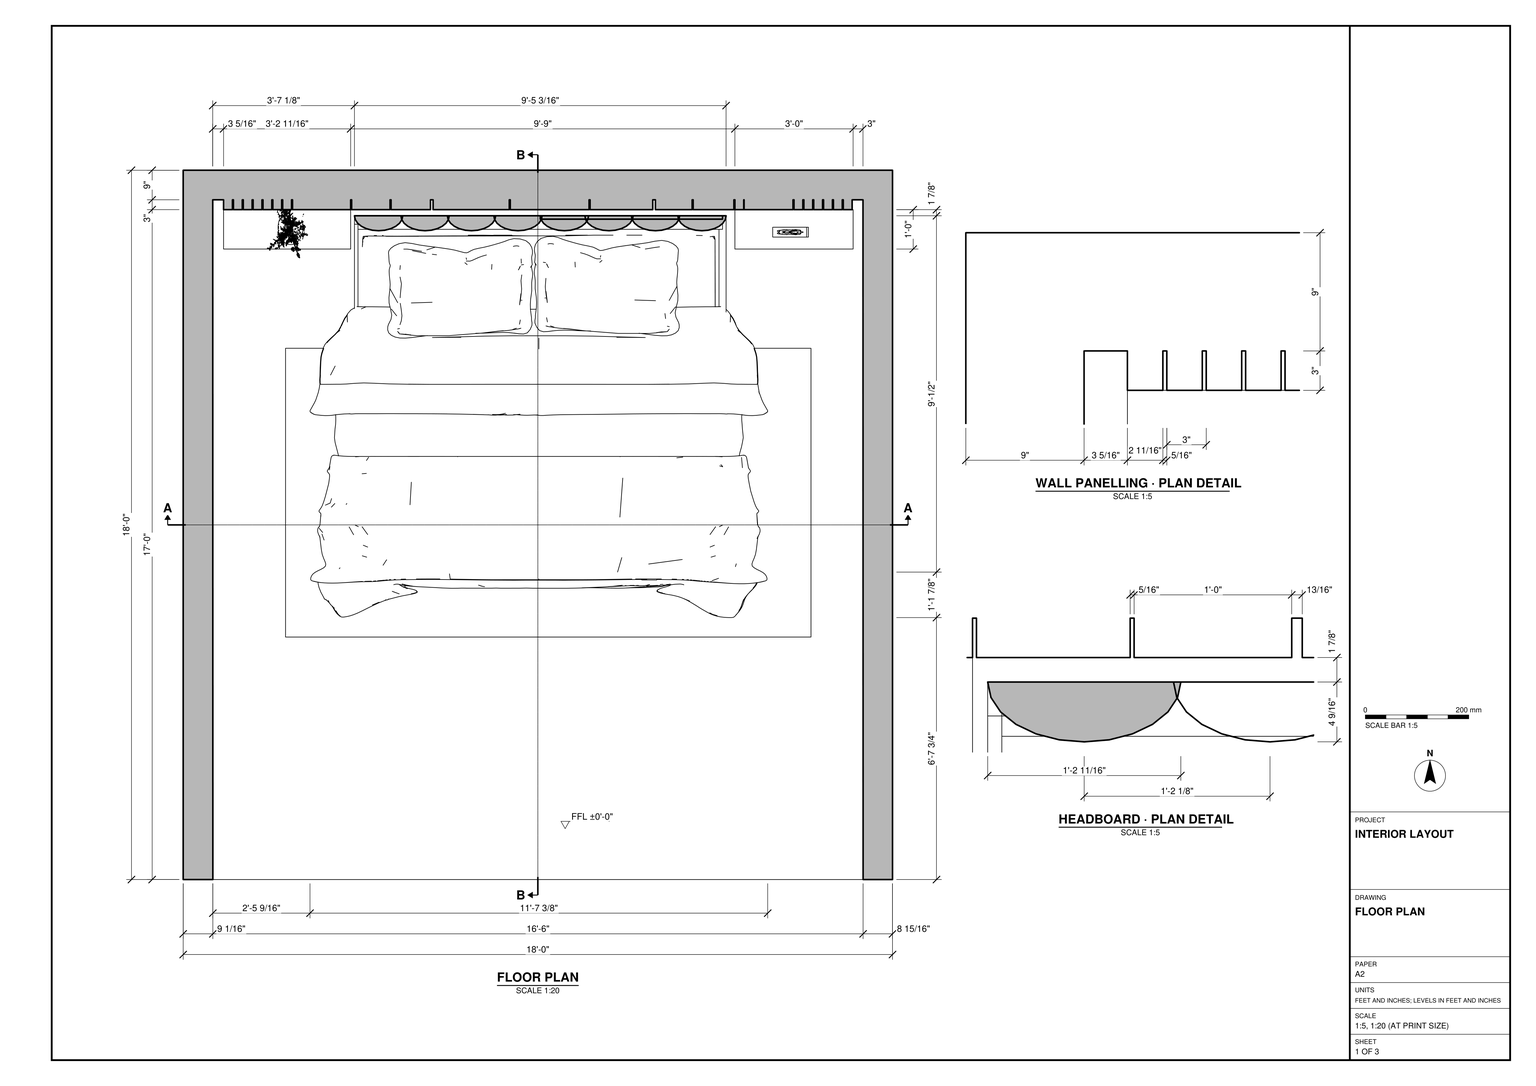
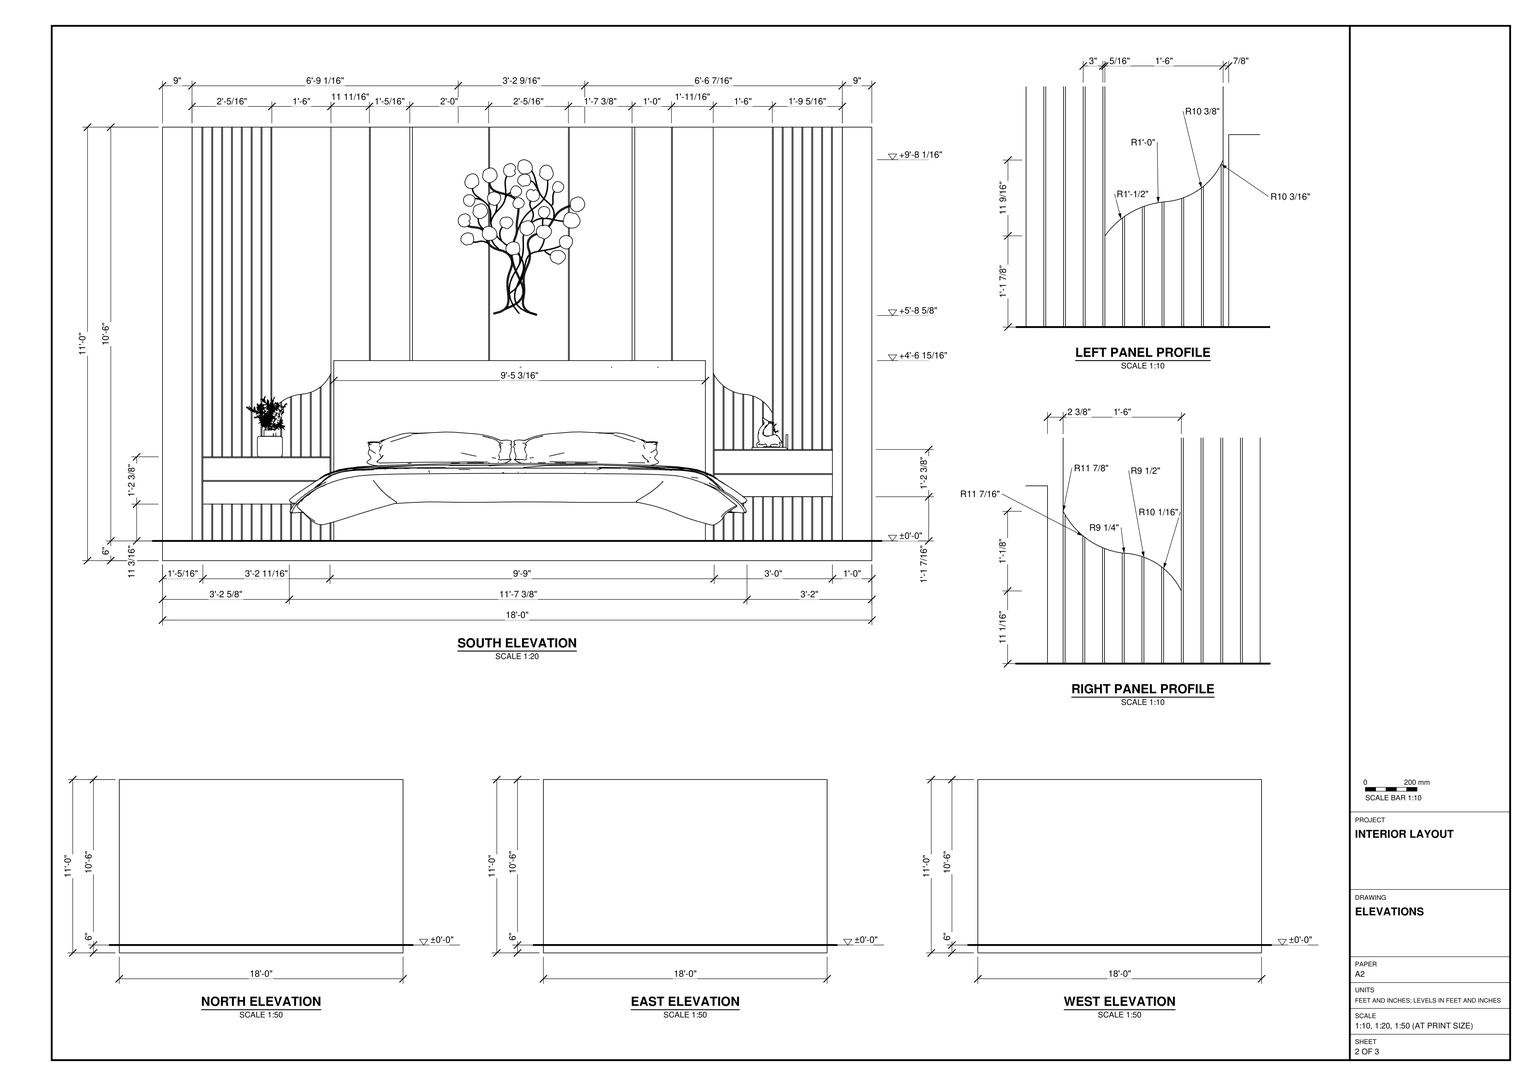
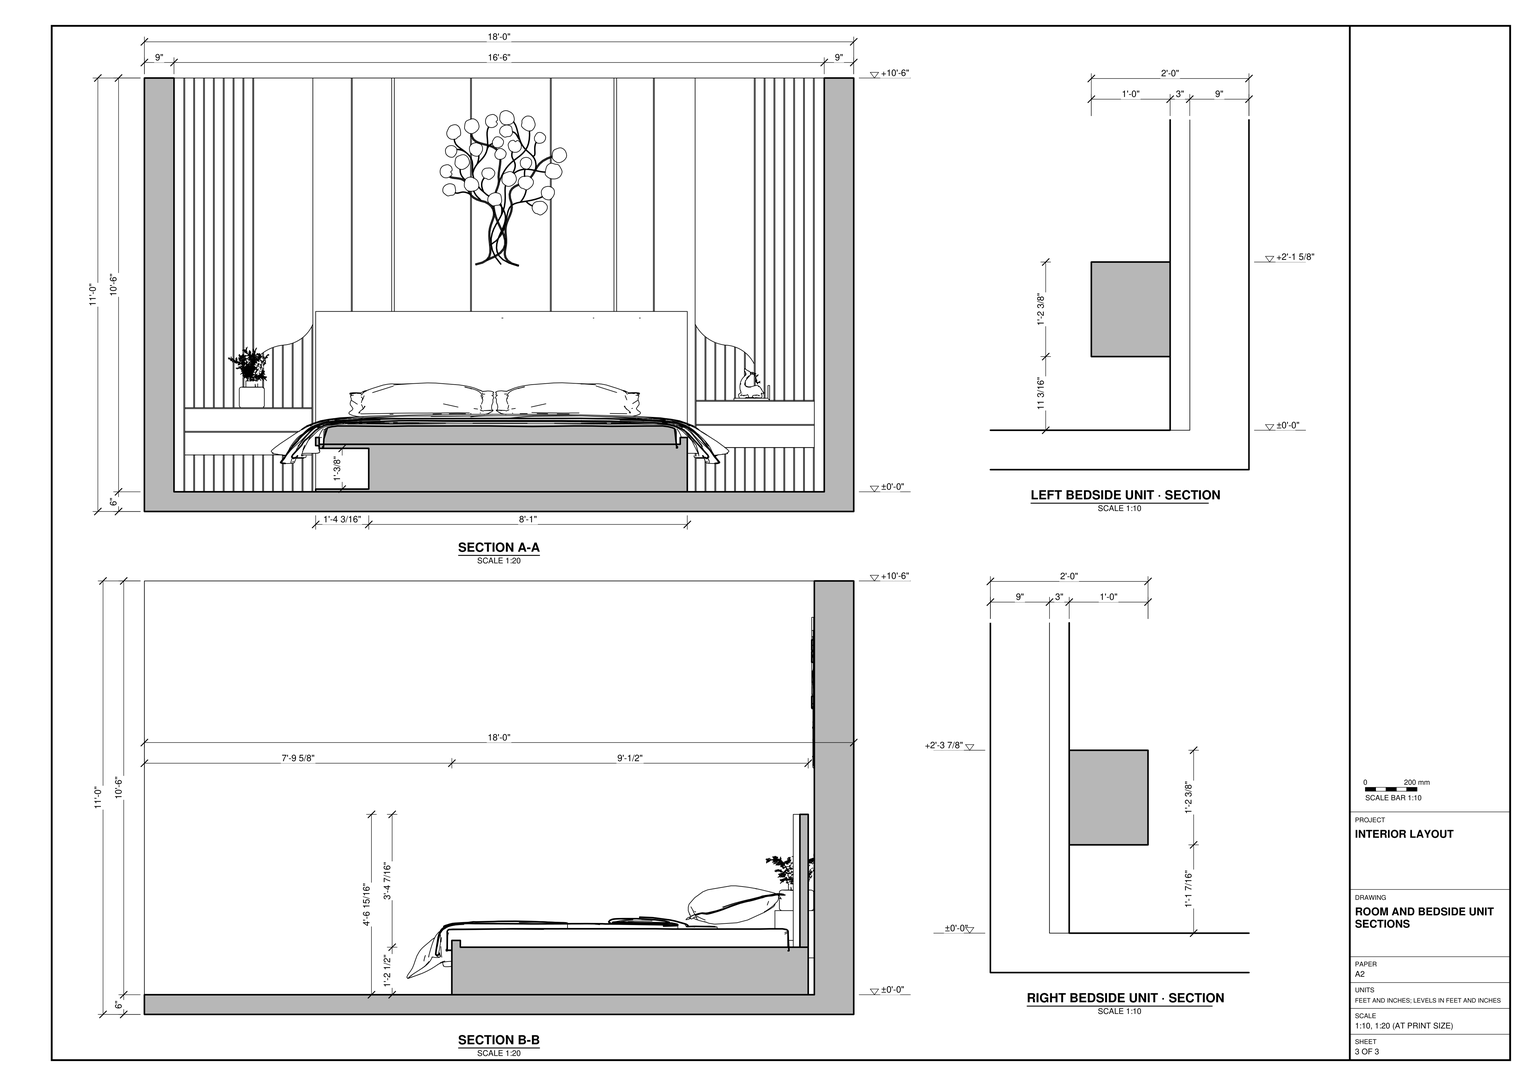
Build the bedroom in SketchUp from task_files/diagram_01.pdf. Work in feet and inches. The room measures 18'-0" by 18'-0" overall and is 11'-0" high from the underside of the floor slab to the wall tops. Set the finished floor at ±0'-0". Model the 6" slab and the three enclosing walls at the thicknesses shown, leaving the side opposite the headboard open as drawn.

Centre the platform bed against the back wall, with the mattress, pillows and covers arranged as in plan. Place the rectangular rug beneath the bed so that it extends beyond the sides and foot. Use the headboard plan detail to form the rounded sections across its face. Behind it, model the broad vertical panels in the middle of the wall and the closely spaced strips toward the ends. Follow the separate left and right profiles where the strip tops curve beside the headboard.

Fit a floating bedside unit on either side of the bed. Use the bedside sections for their projection and mounting heights; the right unit sits slightly higher than the left. Place the wall decoration above the headboard and the small objects on the bedside units as shown. Decor and loose items may be any suitable library components. Keep the walls, slab and each furniture or joinery piece in separate groups or components, and use components for repeated parts. Save one SketchUp model as output_files/bedroom_with_a_panelled_headboard_wall.skp.

# SketchUp Ruby script. Lengths in inches.
U = 1.inch
M = Sketchup.active_model
def pt(a) = Geom::Point3d.new(a.map { |v| v * U })
def face(e, loops, mat)
  f = e.add_face(loops[0].map { |a| pt(a) })
  loops[1..].each { |l| e.add_face(l.map { |a| pt(a) }).erase! }
  f.material = f.back_material = mat if mat
  f
end
# faces: each face lists its corners as indices into pts; further lists are holes
def faces(e, pts, list, mat = nil) = list.each { |f| face(e, (f[0].is_a?(Array) ? f : [f]).map { |l| l.map { |i| pts[i] } }, mat) }
# xy, xz, yz: faces in a plane at the given z, y or x. An outline is a flat list of corners, or four numbers for a rectangle; further outlines are holes
def ring(l) = l.size == 4 ? [[l[0], l[1]], [l[2], l[1]], [l[2], l[3]], [l[0], l[3]]] : l.each_slice(2).to_a
def flat(e, list, mat, &to3) = list.each { |f| face(e, (f[0].is_a?(Array) ? f : [f]).map { |l| ring(l).map { |u, v| to3.(u, v) } }, mat) }
def xy(e, z, list, mat = nil) = flat(e, list, mat) { |x, y| [x, y, z] }
def xz(e, y, list, mat = nil) = flat(e, list, mat) { |x, z| [x, y, z] }
def yz(e, x, list, mat = nil) = flat(e, list, mat) { |y, z| [x, y, z] }
def lines(e, pts, list) = list.each { |a, b| e.add_line(pt(pts[a]), pt(pts[b])) }
# prism: a flat outline (further loops are holes) pulled along v
def prism(e, loops, v, mat = nil)
  f = face(e, loops, mat); d = Geom::Vector3d.new(v.map { |x| x * U })
  f.pushpull(f.normal.samedirection?(d) ? d.length : -d.length)
end
def box(e, o, s, mat = nil) = prism(e, [[o, [o[0] + s[0], o[1], o[2]], [o[0] + s[0], o[1] + s[1], o[2]], [o[0], o[1] + s[1], o[2]]]], [0, 0, s[2]], mat)
def at(x, y, z, deg = 0) = Geom::Transformation.translation(pt([x, y, z])) * Geom::Transformation.rotation(ORIGIN, Z_AXIS, deg.degrees)
def axes(o, x, y, z) = Geom::Transformation.new([*x, 0, *y, 0, *z, 0, *pt(o).to_a, 1])
def part(name) = M.definitions.add(name)
# library, detail: a bought-in or finely detailed component or shape, given as its bounding box
def library(name, o, s) = part(name).tap { |d| box(d.entities, o, s) }
def detail(e, o, s) = box(e.add_group.entities, o, s)
def put(e, d, t, mat = nil) = e.add_instance(d, t).tap { |i| i.material = mat if mat }
def group(e, t, mat = nil) = e.add_group.tap { |g| g.transformation = t; g.material = mat if mat }.entities
root = M.entities
M.materials.add("0890 AP 9857 Lime Burst-N").color = [146, 129, 47]
M.materials.add("W144X914F75_NILAYA EQUINOX FD25701 ROLL F75").color = [234, 241, 241]
M.materials.add("W146Z451B75_NILAYA CITY GLAM 32602 ROLL B75").color = [214, 216, 211]
M.materials.add("[Carpet Berber Pattern Gray]").color = [165, 165, 165]
M.materials.add("[Carrera Marble]").color = [209, 209, 209]
M.materials.add("[Color M03]").color = [170, 170, 170]
M.materials.add("[Wood Veneer 01]").color = [220, 216, 210]
M.materials.add("[Wood Veneer 01]1").color = [220, 216, 210]
M.materials.add("[Wood Veneer 01]2").color = [120, 70, 37]
c1 = library("Group\#96",[6.49,4.72,0.39],[101.82,93.23,52.31])
c2 = library("Group\#9",[0,0,0],[26.76,0.625,32.95])
c3 = library("Agrupar\#3",[0,0,0],[6.2,2.76,4.44])
c4 = library("Group\#168",[-4.85,-5.07,0],[28.06,28.99,27.6])
xy(root,235.32,[[0,0,216,216]])
xy(root,241.32,[[31.17,73.85,191.17,161.78]],"[Carpet Berber Pattern Gray]")
xy(root,241.32,[[[9.04,0,207.04,0,207,207,203.7,207,203.7,204,201,204,201,207,200.7,207,200.7,204,198,204,198,207,197.7,207,197.7,204,195,204,195,207,194.7,207,194.7,204,192,204,192,207,191.7,207,191.7,204,189,204,189,207,188.7,207,188.7,204,186,204,186,207,185.7,207,185.7,204,183,204,183,207,182.7,207,182.7,204,180,204,180,207,179.7,207,179.7,204,177,204,177,207,176.7,207,176.7,204,174,204,174,207,173.7,207,173.7,204,171,204,171,207,170.7,207,170.7,204,168,204,168,207,167.7,207,167.7,204,155.29,204,155.29,207,154.99,207,154.99,204,143.8,204,143.8,207,142.99,207,142.99,204,123.9,204,123.9,207,123.6,207,123.6,204,99.6,204,99.6,207,99.3,207,99.3,204,76.1,204,76.1,207,75.3,207,75.3,204,63.3,204,63.3,207,63,207,63,204,51.3,204,51.3,207,51,207,51,204,48.3,204,48.3,207,48,207,48,204,45.3,204,45.3,207,45,207,45,204,42.3,204,42.3,207,42,207,42,204,39.3,204,39.3,207,39,207,39,204,36.3,204,36.3,207,36,207,36,204,33.3,204,33.3,207,33,207,33,204,30.3,204,30.3,207,30,207,30,204,27.3,204,27.3,207,27,207,27,204,24.3,204,24.3,207,24,207,24,204,21.3,204,21.3,207,21,207,21,204,18.3,204,18.3,207,18,207,18,204,15.3,204,15.3,207,15,207,15,204,12.3,204,12.3,207,9,207],[31.17,73.85,191.17,161.78]]],"[Carrera Marble]")
xy(root,252.54,[[12.3,192,51,204]])
xy(root,254.77,[[168,192,204,204]])
xy(root,266.9375,[[12.3,192,51,204]])
xy(root,269.17,[[168,192,204,204]])
xy(root,367.32,[[0,0,9.04,0,9,207,12.3,207,12.3,204,15,204,15,207,15.3,207,15.3,204,18,204,18,207,18.3,207,18.3,204,21,204,21,207,21.3,207,21.3,204,24,204,24,207,24.3,207,24.3,204,27,204,27,207,27.3,207,27.3,204,30,204,30,207,30.3,207,30.3,204,33,204,33,207,33.3,207,33.3,204,63,204,63,207,63.3,207,63.3,204,75.3,204,75.3,207,76.1,207,76.1,204,99.3,204,99.3,207,99.6,207,99.6,204,123.6,204,123.6,207,123.9,207,123.9,204,142.99,204,142.99,207,143.8,207,143.8,204,154.99,204,154.99,207,155.29,207,155.29,204,167.7,204,167.7,207,186,207,186,204,188.7,204,188.7,207,189,207,189,204,191.7,204,191.7,207,192,207,192,204,194.7,204,194.7,207,195,207,195,204,197.7,204,197.7,207,198,207,198,204,200.7,204,200.7,207,201,207,201,204,203.7,204,203.7,207,207,207,207.04,0,216,0,216,216,0,216],[167.7,204,185.7,207]])
xz(root,0,[[0,235.32,216,235.32,216,367.32,207.04,367.32,207.04,241.32,9.04,241.32,9.04,367.32,0,367.32]])
xz(root,192,[[12.3,252.54,51,259.4375],[168,254.77,204,254.81],[168,254.81,204,261.54],[12.3,259.4375,51,259.74],[12.3,259.74,51,266.64],
  [168,261.54,204,261.84],[168,261.84,204,268.87],[12.3,266.64,51,266.9375],[168,268.87,204,269.17]])
xz(root,204,[[15,252.54,15.3,266.9375],[18,252.54,18.3,266.9375],[21,252.54,21.3,266.9375],[24,252.54,24.3,266.9375],[27,252.54,27.3,266.9375],
  [30,252.54,30.3,266.9375],[33,252.54,33.3,266.9375],[36,252.54,36.3,266.9375],[39,252.54,39.3,266.9375],[42,252.54,42.3,266.9375],
  [45,252.54,45.3,266.9375],[48,252.54,48.3,266.9375],[170.7,254.77,171,269.17],[173.7,254.77,174,269.17],[176.7,254.77,177,269.17],
  [179.7,254.77,180,269.17],[182.7,254.77,183,269.17],[185.7,254.77,186,269.17],[188.7,254.77,189,269.17],[191.7,254.77,192,269.17],
  [194.7,254.77,195,269.17],[197.7,254.77,198,269.17],[200.7,254.77,201,269.17],[203.7,254.77,204,269.17]])
xz(root,204,[[51.3,241.32,63,367.32],[63.3,241.32,75.3,367.32],[76.1,241.32,99.3,367.32],[99.6,241.32,123.6,367.32],[123.9,241.32,142.99,367.32],
  [143.8,241.32,154.99,367.32],[155.29,241.32,167.7,367.32]],"[Color M03]")
xz(root,204,[[33.3,280.83,33.85,281.54,34.4375,282.2,35.08,282.82,35.76,283.39,36,283.57,36.3,283.79,36.48,283.92,37.24,284.39,38.03,284.8,38.84,285.16,39,285.22,39.3,285.33,39.68,285.46,40.54,285.7,41.42,285.88,42,285.96,42.3,286,43.26,286.1,44.21,286.3,45,286.53,45.14,286.58,45.3,286.64,46.03,286.94,46.89,287.39,47.71,287.91,48,288.14,48.3,288.37,48.47,288.5,49.17,289.17,49.81,289.89,50.39,290.67,50.88,291.51,51,291.75,51.3,292.38,51.3,367.32,33.3,367.32]],"[Wood Veneer 01]")
xz(root,204,[[185.7,280.23,185.7,367.32,167.7,367.32,167.7,292.38,168,291.85,168.17,291.55,168.7,290.76,169.3,290.01,169.95,289.3125,170.66,288.67,170.7,288.64,171,288.41,171.42,288.09,172.22,287.57,173.06,287.11,173.7,286.83,173.93,286.73,174,286.71,174.84,286.41,175.76,286.17,176.7,286.01,177,285.99,177.63,285.94,178.56,285.79,179.47,285.56,179.7,285.48,180,285.37,180.35,285.25,181.2,284.85,182.01,284.38,182.7,283.89,182.77,283.84,183,283.65,183.49,283.23,184.14,282.5625,184.73,281.84,185.25,281.06]],"[Wood Veneer 01]1")
xz(root,204,[[12.3,241.32,15,252.54],[15.3,241.32,18,252.54],[18.3,241.32,21,252.54],[21.3,241.32,24,252.54],[24.3,241.32,27,252.54],
  [27.3,241.32,30,252.54],[30.3,241.32,33,252.54],[33.3,241.32,36,252.54],[36.3,241.32,39,252.54],[39.3,241.32,42,252.54],
  [42.3,241.32,45,252.54],[45.3,241.32,48,252.54],[48.3,241.32,51,252.54],[168,241.32,170.7,254.77],[171,241.32,173.7,254.77],
  [174,241.32,176.7,254.77],[177,241.32,179.7,254.77],[180,241.32,182.7,254.77],[183,241.32,185.7,254.77],[186,241.32,188.7,254.77],
  [189,241.32,191.7,254.77],[192,241.32,194.7,254.77],[195,241.32,197.7,254.77],[198,241.32,200.7,254.77],[201,241.32,203.7,254.77],
  [12.3,252.54,15,266.9375],[15.3,252.54,18,266.9375],[18.3,252.54,21,266.9375],[21.3,252.54,24,266.9375],[24.3,252.54,27,266.9375],
  [27.3,252.54,30,266.9375],[30.3,252.54,33,266.9375],[33.3,252.54,36,266.9375],[36.3,252.54,39,266.9375],[39.3,252.54,42,266.9375],
  [42.3,252.54,45,266.9375],[45.3,252.54,48,266.9375],[48.3,252.54,51,266.9375],[168,254.77,170.7,269.17],[171,254.77,173.7,269.17],
  [174,254.77,176.7,269.17],[177,254.77,179.7,269.17],[180,254.77,182.7,269.17],[183,254.77,185.7,269.17],[186,254.77,188.7,269.17],
  [189,254.77,191.7,269.17],[192,254.77,194.7,269.17],[195,254.77,197.7,269.17],[198,254.77,200.7,269.17],[201,254.77,203.7,269.17],
  [12.3,266.9375,15,367.32],[15.3,266.9375,18,367.32],[18.3,266.9375,21,367.32],[21.3,266.9375,24,367.32],[24.3,266.9375,27,367.32],
  [27.3,266.9375,30,367.32],[30.3,266.9375,33,367.32],[33.3,266.9375,36,266.9375,36,283.57,35.76,283.39,35.08,282.82,34.4375,282.2,33.85,281.54,33.3,280.83],[36.3,266.9375,39,266.9375,39,285.22,38.84,285.16,38.03,284.8,37.24,284.39,36.48,283.92,36.3,283.79],[39.3,266.9375,42,266.9375,42,285.96,41.42,285.88,40.54,285.7,39.68,285.46,39.3,285.33],
  [42.3,266.9375,45,266.9375,45,286.53,44.21,286.3,43.26,286.1,42.3,286],[45.3,266.9375,48,266.9375,48,288.14,47.71,287.91,46.89,287.39,46.03,286.94,45.3,286.64],[48.3,266.9375,51,266.9375,51,291.75,50.88,291.51,50.39,290.67,49.81,289.89,49.17,289.17,48.47,288.5,48.3,288.37],[168,269.17,170.7,269.17,170.7,288.64,170.66,288.67,169.95,289.3125,169.3,290.01,168.7,290.76,168.17,291.55,168,291.85],[171,269.17,173.7,269.17,173.7,286.83,173.06,287.11,172.22,287.57,171.42,288.09,171,288.41],
  [174,269.17,176.7,269.17,176.7,286.01,175.76,286.17,174.84,286.41,174,286.71],[177,269.17,179.7,269.17,179.7,285.48,179.47,285.56,178.56,285.79,177.63,285.94,177,285.99],[180,269.17,182.7,269.17,182.7,283.89,182.01,284.38,181.2,284.85,180.35,285.25,180,285.37],[183,269.17,185.7,269.17,185.7,280.23,185.25,281.06,184.73,281.84,184.14,282.5625,183.49,283.23,183,283.65],[186,269.17,188.7,367.32],
  [189,269.17,191.7,367.32],[192,269.17,194.7,367.32],[195,269.17,197.7,367.32],[198,269.17,200.7,367.32],[201,269.17,203.7,367.32]],"[Wood Veneer 01]2")
xz(root,207,[[9,241.32,12,367.32],[12,241.32,12.3,367.32],[15,241.32,15.3,367.32],[18,241.32,18.3,367.32],[21,241.32,21.3,367.32],
  [24,241.32,24.3,367.32],[27,241.32,27.3,367.32],[30,241.32,30.3,367.32],[33,241.32,33.3,367.32],[36,241.32,36.3,241.32,36.3,283.79,36,283.57],
  [39,241.32,39.3,241.32,39.3,285.33,39,285.22],[42,241.32,42.3,241.32,42.3,286,42,285.96],[48,241.32,48.3,241.32,48.3,288.37,48,288.14],[51,241.32,51.3,241.32,51.3,292.38,51,291.75],[63,241.32,63.3,367.32],
  [99.3,241.32,99.6,367.32],[123.6,241.32,123.9,367.32],[154.99,241.32,155.29,367.32],[167.7,241.32,168,241.32,168,291.85,167.7,292.38],[170.7,241.32,171,241.32,171,288.41,170.7,288.64],
  [173.7,241.32,174,241.32,174,286.71,173.93,286.73,173.7,286.83],[176.7,241.32,177,241.32,177,285.99,176.7,286.01],[179.7,241.32,180,241.32,180,285.37,179.7,285.48],[182.7,241.32,183,241.32,183,283.65,182.77,283.84,182.7,283.89],[185.7,241.32,186,367.32],
  [188.7,241.32,189,367.32],[191.7,241.32,192,367.32],[194.7,241.32,195,367.32],[197.7,241.32,198,367.32],[200.7,241.32,201,367.32],
  [203.7,241.32,204,367.32],[204,241.32,207,367.32]])
xz(root,207,[[75.3,241.32,76.1,367.32],[142.99,241.32,143.8,367.32]],"0890 AP 9857 Lime Burst-N")
xz(root,216,[[0,235.32,216,367.32]])
yz(root,0,[[0,235.32,216,367.32]])
yz(root,12.3,[[204,241.32,207,367.32],[192,252.54,204,266.9375]])
yz(root,15,[[204,241.32,207,367.32]])
yz(root,15.3,[[204,241.32,207,367.32]])
yz(root,18,[[204,241.32,207,367.32]])
yz(root,18.3,[[204,241.32,207,367.32]])
yz(root,21,[[204,241.32,207,367.32]])
yz(root,21.3,[[204,241.32,207,367.32]])
yz(root,24,[[204,241.32,207,367.32]])
yz(root,24.3,[[204,241.32,207,367.32]])
yz(root,27,[[204,241.32,207,367.32]])
yz(root,27.3,[[204,241.32,207,367.32]])
yz(root,30,[[204,241.32,207,367.32]])
yz(root,30.3,[[204,241.32,207,367.32]])
yz(root,33,[[204,241.32,207,367.32]])
yz(root,33.3,[[204,241.32,207,280.83],[204,280.83,207,367.32]])
yz(root,36,[[204,241.32,207,283.57]])
yz(root,36.3,[[204,241.32,207,283.79]])
yz(root,39,[[204,241.32,207,285.22]])
yz(root,39.3,[[204,241.32,207,285.33]])
yz(root,42,[[204,241.32,207,285.96]])
yz(root,42.3,[[204,241.32,207,286]])
yz(root,45.3,[[204,241.32,207,286.64]])
yz(root,48,[[204,241.32,207,288.14]])
yz(root,48.3,[[204,241.32,207,288.37]])
yz(root,51,[[204,241.32,207,291.75],[192,252.54,204,266.9375]])
yz(root,51.3,[[204,241.32,207,292.38]],"[Color M03]")
yz(root,63,[[204,241.32,207,367.32]],"[Color M03]")
yz(root,63.3,[[204,241.32,207,367.32]],"[Color M03]")
yz(root,75.3,[[204,241.32,207,367.32]],"[Color M03]")
yz(root,76.1,[[204,241.32,207,367.32]],"[Color M03]")
yz(root,99.3,[[204,241.32,207,367.32]],"[Color M03]")
yz(root,99.6,[[204,241.32,207,367.32]],"[Color M03]")
yz(root,123.6,[[204,241.32,207,367.32]],"[Color M03]")
yz(root,123.9,[[204,241.32,207,367.32]],"[Color M03]")
yz(root,142.99,[[204,241.32,207,367.32]],"[Color M03]")
yz(root,143.8,[[204,241.32,207,367.32]],"[Color M03]")
yz(root,154.99,[[204,241.32,207,367.32]],"[Color M03]")
yz(root,155.29,[[204,241.32,207,367.32]],"[Color M03]")
yz(root,167.7,[[204,241.32,207,292.38]],"[Color M03]")
yz(root,168,[[204,241.32,207,291.85],[192,254.77,204,269.17]])
yz(root,170.7,[[204,241.32,207,288.64]])
yz(root,171,[[204,241.32,207,288.41]])
yz(root,173.7,[[204,241.32,207,286.83]])
yz(root,174,[[204,241.32,207,286.71]])
yz(root,176.7,[[204,241.32,207,286.01]])
yz(root,177,[[204,241.32,207,285.99]])
yz(root,179.7,[[204,241.32,207,285.48]])
yz(root,180,[[204,241.32,207,285.37]])
yz(root,182.7,[[204,241.32,207,283.89]])
yz(root,183,[[204,241.32,207,283.65]])
yz(root,185.7,[[204,241.32,207,280.23],[204,280.23,207,367.32]])
yz(root,186,[[204,241.32,207,367.32]])
yz(root,188.7,[[204,241.32,207,367.32]])
yz(root,189,[[204,241.32,207,367.32]])
yz(root,191.7,[[204,241.32,207,367.32]])
yz(root,192,[[204,241.32,207,367.32]])
yz(root,194.7,[[204,241.32,207,367.32]])
yz(root,195,[[204,241.32,207,367.32]])
yz(root,197.7,[[204,241.32,207,367.32]])
yz(root,198,[[204,241.32,207,367.32]])
yz(root,200.7,[[204,241.32,207,367.32]])
yz(root,201,[[204,241.32,207,367.32]])
yz(root,203.7,[[204,241.32,207,367.32]])
yz(root,204,[[192,254.77,204,269.17]])
yz(root,216,[[0,235.32,216,367.32]])
p = [[9.04,0,241.32],[9,207,241.32],[9,207,367.32],[9.04,0,367.32],[207,207,241.32],[207.04,0,241.32],
  [207.04,0,367.32],[207,207,367.32],[36.3,204,283.79],[36,204,283.57],[36,207,283.57],[36.3,207,283.79],
  [182.77,207,283.84],[183,207,283.65],[183,204,283.65],[182.77,204,283.84],[182.7,207,283.89],[182.7,204,283.89],
  [39.3,204,285.33],[39,204,285.22],[39,207,285.22],[39.3,207,285.33],[179.7,207,285.48],[180,207,285.37],
  [180,204,285.37],[179.7,204,285.48],[42.3,204,286],[42,204,285.96],[42,207,285.96],[42.3,207,286],
  [176.7,207,286.01],[177,207,285.99],[177,204,285.99],[176.7,204,286.01],[45.14,204,286.58],[45,204,286.53],
  [45,207,286.53],[45.14,207,286.58],[45.3,207,286.64],[45.3,204,286.64],[173.7,207,286.83],[173.93,207,286.73],
  [173.93,204,286.73],[173.7,204,286.83],[174,207,286.71],[174,204,286.71],[48.3,204,288.37],[48,204,288.14],
  [48,207,288.14],[48.3,207,288.37],[170.7,207,288.64],[171,207,288.41],[171,204,288.41],[170.7,204,288.64],
  [51.3,204,292.38],[51,204,291.75],[51,207,291.75],[51.3,207,292.38],[167.7,207,292.38],[168,207,291.85],
  [168,204,291.85],[167.7,204,292.38],[48,207,288.37],[45,207,286.64],[51,207,292.38],[36,207,283.79],
  [39,207,285.33],[42,207,286]]
faces(root,p,[[0,1,2,3]],"W144X914F75_NILAYA EQUINOX FD25701 ROLL F75")
faces(root,p,[[4,5,6,7]],"W146Z451B75_NILAYA CITY GLAM 32602 ROLL B75")
faces(root,p,[[8,9,10,11],[12,13,14,15],[16,12,15,17],[18,19,20,21],[22,23,24,25],[26,27,28,29],[30,31,32,33],[34,35,36,37],
  [37,38,39,34],[40,41,42,43],[41,44,45,42],[46,47,48,49],[50,51,52,53],[54,55,56,57],[58,59,60,61]])
lines(root,p,[[48,62],[36,63],[56,64],[10,65],[20,66],[28,67]])
put(root,c1,axes([186.875,208.34,240.91],[-1.36876,0,0],[0,-1.3125,0],[0,0,1.05]))
put(root,c2,axes([90.04,203.1,309.96],[1.44,0,0],[0,1.44,0],[0,0,1.44]))
put(root,c3,axes([179.51,195.64,269.17],[1.75534,0,0],[0,1.09,0],[0,0,2.18]))
put(root,c4,axes([25.53,189.27,266.9375],[0.73124,0,0],[0,1,0],[0,0,0.67]))
